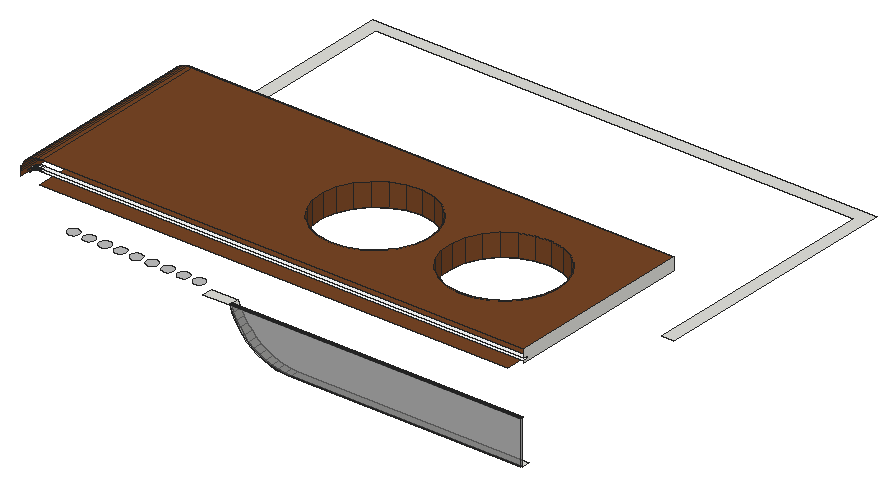
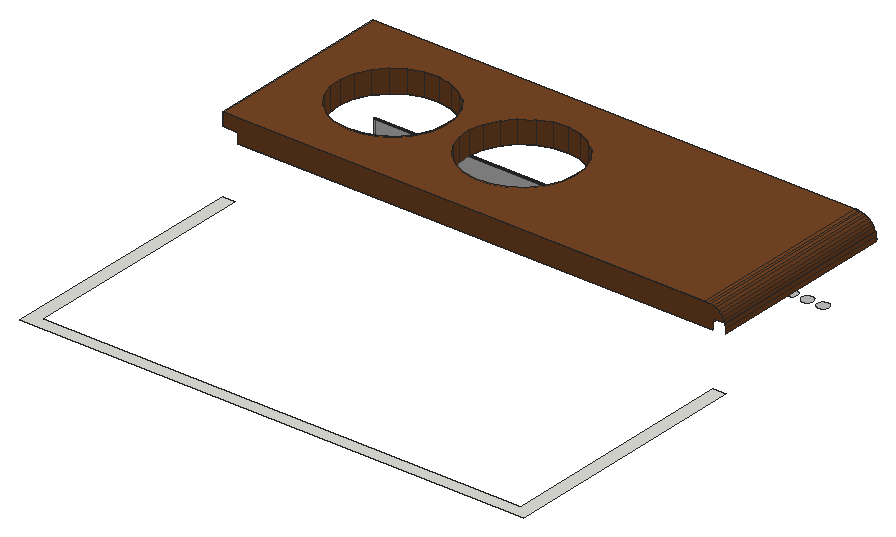
# SketchUp Ruby script. Lengths in millimetres.
U = 1.mm
M = Sketchup.active_model
def pt(a) = Geom::Point3d.new(a.map { |v| v * U })
def face(e, loops, mat)
  f = e.add_face(loops[0].map { |a| pt(a) })
  loops[1..].each { |l| e.add_face(l.map { |a| pt(a) }).erase! }
  f.material = f.back_material = mat if mat
  f
end
# faces: each face lists its corners as indices into pts; further lists are holes
def faces(e, pts, list, mat = nil) = list.each { |f| face(e, (f[0].is_a?(Array) ? f : [f]).map { |l| l.map { |i| pts[i] } }, mat) }
# xy, xz, yz: faces in a plane at the given z, y or x. An outline is a flat list of corners, or four numbers for a rectangle; further outlines are holes
def ring(l) = l.size == 4 ? [[l[0], l[1]], [l[2], l[1]], [l[2], l[3]], [l[0], l[3]]] : l.each_slice(2).to_a
def flat(e, list, mat, &to3) = list.each { |f| face(e, (f[0].is_a?(Array) ? f : [f]).map { |l| ring(l).map { |u, v| to3.(u, v) } }, mat) }
def xy(e, z, list, mat = nil) = flat(e, list, mat) { |x, y| [x, y, z] }
def xz(e, y, list, mat = nil) = flat(e, list, mat) { |x, z| [x, y, z] }
def yz(e, x, list, mat = nil) = flat(e, list, mat) { |y, z| [x, y, z] }
def lines(e, pts, list) = list.each { |a, b| e.add_line(pt(pts[a]), pt(pts[b])) }
# prism: a flat outline (further loops are holes) pulled along v
def prism(e, loops, v, mat = nil)
  f = face(e, loops, mat); d = Geom::Vector3d.new(v.map { |x| x * U })
  f.pushpull(f.normal.samedirection?(d) ? d.length : -d.length)
end
def box(e, o, s, mat = nil) = prism(e, [[o, [o[0] + s[0], o[1], o[2]], [o[0] + s[0], o[1] + s[1], o[2]], [o[0], o[1] + s[1], o[2]]]], [0, 0, s[2]], mat)
def at(x, y, z, deg = 0) = Geom::Transformation.translation(pt([x, y, z])) * Geom::Transformation.rotation(ORIGIN, Z_AXIS, deg.degrees)
def axes(o, x, y, z) = Geom::Transformation.new([*x, 0, *y, 0, *z, 0, *pt(o).to_a, 1])
def part(name) = M.definitions.add(name)
# library, detail: a bought-in or finely detailed component or shape, given as its bounding box
def library(name, o, s) = part(name).tap { |d| box(d.entities, o, s) }
def detail(e, o, s) = box(e.add_group.entities, o, s)
def put(e, d, t, mat = nil) = e.add_instance(d, t).tap { |i| i.material = mat if mat }
def group(e, t, mat = nil) = e.add_group.tap { |g| g.transformation = t; g.material = mat if mat }.entities
root = M.entities
M.materials.add("[Color M00]").color = [255, 255, 255]
M.materials.add("[Color M07]").color = [58, 58, 58]
M.materials.add("[Metal Corrugated Shiny]").color = [193, 193, 193]
M.materials.add("[Translucent Glass Gray]").color = [128, 128, 128]
M.materials["[Translucent Glass Gray]"].alpha = 0.5
M.materials.add("[Wood Veneer 01]").color = [120, 70, 37]
xy(root,7765.4,[[6213.6,642.9,11814.3,849.3]])
xy(root,7765.4,[[6213.6,582.5,11814.3,606.3],[6213.6,606.3,11814.3,642.9]],"[Translucent Glass Gray]")
xy(root,8813.8,[[4124.5,582.5,4764.3,849.3],[3.3,4760.9,308.1,4760.9,308.1,10572.8,11890.5,10572.8,11890.5,4760.9,12195.3,4760.9,12195.3,10877.6,3.3,10877.6]])
xy(root,8813.8,[[4764.3,606.3,11814.3,642.9]],"[Color M07]")
xy(root,8813.8,[[696.7,818.4,730.8,823.2,762.4,836.7,789.5,858,810.2,885.5,823,917.4,827.1,951.5,822.3,985.6,808.8,1017.2,787.6,1044.3,760.1,1064.9,728.2,1077.8,694,1081.9,660,1077.1,628.3,1063.6,601.3,1042.4,580.6,1014.9,567.8,983,563.6,948.8,568.5,914.8,582,883.1,603.2,856,630.7,835.4,662.6,822.5],[1077.7,818.4,1111.8,823.2,1143.4,836.7,1170.5,858,1191.2,885.5,1204,917.4,1208.1,951.5,1203.3,985.6,1189.8,1017.2,1168.6,1044.3,1141.1,1064.9,1109.2,1077.8,1075,1081.9,1041,1077.1,1009.3,1063.6,982.3,1042.4,961.6,1014.9,948.8,983,944.6,948.8,949.5,914.8,963,883.1,984.2,856,1011.7,835.4,1043.6,822.5],[1458.7,818.4,1492.8,823.2,1524.4,836.7,1551.5,858,1572.2,885.5,1585,917.4,1589.1,951.5,1584.3,985.6,1570.8,1017.2,1549.6,1044.3,1522.1,1064.9,1490.2,1077.8,1456,1081.9,1422,1077.1,1390.3,1063.6,1363.3,1042.4,1342.6,1014.9,1329.8,983,1325.6,948.8,1330.5,914.8,1344,883.1,1365.2,856,1392.7,835.4,1424.6,822.5],[1839.7,818.4,1873.8,823.2,1905.4,836.7,1932.5,858,1953.2,885.5,1966,917.4,1970.1,951.5,1965.3,985.6,1951.8,1017.2,1930.6,1044.3,1903.1,1064.9,1871.2,1077.8,1837,1081.9,1803,1077.1,1771.3,1063.6,1744.3,1042.4,1723.6,1014.9,1710.8,983,1706.6,948.8,1711.5,914.8,1725,883.1,1746.2,856,1773.7,835.4,1805.6,822.5],[2220.7,818.4,2254.8,823.2,2286.4,836.7,2313.5,858,2334.2,885.5,2347,917.4,2351.1,951.5,2346.3,985.6,2332.8,1017.2,2311.6,1044.3,2284.1,1064.9,2252.2,1077.8,2218,1081.9,2184,1077.1,2152.3,1063.6,2125.3,1042.4,2104.6,1014.9,2091.8,983,2087.6,948.8,2092.5,914.8,2106,883.1,2127.2,856,2154.7,835.4,2186.6,822.5],
  [2601.7,818.4,2635.8,823.2,2667.4,836.7,2694.5,858,2715.2,885.5,2728,917.4,2732.1,951.5,2727.3,985.6,2713.8,1017.2,2692.6,1044.3,2665.1,1064.9,2633.2,1077.8,2599,1081.9,2565,1077.1,2533.3,1063.6,2506.3,1042.4,2485.6,1014.9,2472.8,983,2468.6,948.8,2473.5,914.8,2487,883.1,2508.2,856,2535.7,835.4,2567.6,822.5],[2982.7,818.4,3016.8,823.2,3048.4,836.7,3075.5,858,3096.2,885.5,3109,917.4,3113.1,951.5,3108.3,985.6,3094.8,1017.2,3073.6,1044.3,3046.1,1064.9,3014.2,1077.8,2980,1081.9,2946,1077.1,2914.3,1063.6,2887.3,1042.4,2866.6,1014.9,2853.8,983,2849.6,948.8,2854.5,914.8,2868,883.1,2889.2,856,2916.7,835.4,2948.6,822.5],[3363.7,818.4,3397.8,823.2,3429.4,836.7,3456.5,858,3477.2,885.5,3490,917.4,3494.1,951.5,3489.3,985.6,3475.8,1017.2,3454.6,1044.3,3427.1,1064.9,3395.2,1077.8,3361,1081.9,3327,1077.1,3295.3,1063.6,3268.3,1042.4,3247.6,1014.9,3234.8,983,3230.6,948.8,3235.5,914.8,3249,883.1,3270.2,856,3297.7,835.4,3329.6,822.5],[3744.7,818.4,3778.8,823.2,3810.4,836.7,3837.5,858,3858.2,885.5,3871,917.4,3875.1,951.5,3870.3,985.6,3856.8,1017.2,3835.6,1044.3,3808.1,1064.9,3776.2,1077.8,3742,1081.9,3708,1077.1,3676.3,1063.6,3649.3,1042.4,3628.6,1014.9,3615.8,983,3611.6,948.8,3616.5,914.8,3630,883.1,3651.2,856,3678.7,835.4,3710.6,822.5]],"[Metal Corrugated Shiny]")
xy(root,8839.2,[[4764.3,606.3,11814.3,642.9]],"[Color M07]")
xy(root,10096.5,[[[479.5,209.6,11814.3,4760.9],[9848.2,1135,10193.1,1163.4,10518.9,1280.1,10803.4,1477.1,11027.2,1741,11175.1,2053.9,11236.9,2394.3,11208.5,2739.2,11091.9,3065,10894.9,3349.5,10630.9,3573.3,10318.1,3721.2,9977.6,3783,9632.7,3754.6,9307,3638,9022.5,3441,8798.7,3177,8650.8,2864.2,8588.9,2523.7,8617.3,2178.8,8734,1853.1,8931,1568.6,9194.9,1344.8,9507.8,1196.9],[6725.6,1135,7070.5,1163.4,7396.3,1280.1,7680.8,1477.1,7904.6,1741,8052.4,2053.9,8114.3,2394.3,8085.9,2739.2,7969.3,3065,7772.3,3349.5,7508.3,3573.3,7195.5,3721.2,6855,3783,6510.1,3754.6,6184.4,3638,5899.9,3441,5676.1,3177,5528.2,2864.2,5466.3,2523.7,5494.7,2178.8,5611.4,1853.1,5808.4,1568.6,6072.3,1344.8,6385.2,1196.9]]],"[Wood Veneer 01]")
xy(root,10388.1,[[531,209.6,12195.3,325.4]],"[Color M00]")
xy(root,10446.7,[[531,209.6,12195.3,325.4]],"[Color M00]")
xy(root,10642.6,[[432,209.6,511.9,4760.9],[[511.9,209.6,12195.3,4760.9],[6725.6,1135,6385.2,1196.9,6072.3,1344.8,5808.4,1568.6,5611.4,1853.1,5494.7,2178.8,5466.3,2523.7,5528.2,2864.2,5676.1,3177,5899.9,3441,6184.4,3638,6510.1,3754.6,6855,3783,7195.5,3721.2,7508.3,3573.3,7772.3,3349.5,7969.3,3065,8085.9,2739.2,8114.3,2394.3,8052.4,2053.9,7904.6,1741,7680.8,1477.1,7396.3,1280.1,7070.5,1163.4],[9848.2,1135,9507.8,1196.9,9194.9,1344.8,8931,1568.6,8734,1853.1,8617.3,2178.8,8588.9,2523.7,8650.8,2864.2,8798.7,3177,9022.5,3441,9307,3638,9632.7,3754.6,9977.6,3783,10318.1,3721.2,10630.9,3573.3,10894.9,3349.5,11091.9,3065,11208.5,2739.2,11236.9,2394.3,11175.1,2053.9,11027.2,1741,10803.4,1477.1,10518.9,1280.1,10193.1,1163.4]]],"[Wood Veneer 01]")
xz(root,209.6,[[3.3,10119.6,3.3,10221.2,0,10189.2],[432,10642.6,511.9,10642.6,442.3,10643.9]])
xz(root,606.3,[[4764.3,8813.8,11814.3,8839.2]],"[Color M07]")
xz(root,606.3,[[6213.6,7765.4,11814.3,7765.4,11814.3,8813.8,4764.3,8813.8,4822,8665.4,4894.7,8523.8,4981.9,8390.6,5082.4,8267.2,5195.3,8154.9,5319.2,8055,5452.9,7968.5,5594.8,7896.5,5743.5,7839.6,5897.3,7798.5,6054.6,7773.7]],"[Translucent Glass Gray]")
xz(root,642.9,[[4764.3,8813.8,11814.3,8839.2]],"[Color M07]")
xz(root,642.9,[[6213.6,7765.4,6054.6,7773.7,5897.3,7798.5,5743.5,7839.6,5594.8,7896.5,5452.9,7968.5,5319.2,8055,5195.3,8154.9,5082.4,8267.2,4981.9,8390.6,4894.7,8523.8,4822,8665.4,4764.3,8813.8,11814.3,8813.8,11814.3,7765.4]],"[Translucent Glass Gray]")
xz(root,4760.9,[[3.3,10221.2,3.3,10337.8,29.4,10337.8,24.3,10325.9,7.1,10258.4]])
xz(root,4760.9,[[308.1,10096.5,308.1,10337.8,29.4,10337.8,51.4,10390.1,87.7,10449.5,132.4,10502.9,184.5,10549,242.9,10587,306.3,10615.8,373.3,10634.9,432,10642.6,12195.3,10642.6,12195.3,10337.8,11814.3,10337.8,11814.3,10096.5]],"[Wood Veneer 01]")
yz(root,3.3,[[209.6,10119.6,4760.9,10221.2],[209.6,10221.2,4760.9,10337.8]],"[Wood Veneer 01]")
yz(root,4764.3,[[606.3,8813.8,642.9,8839.2]],"[Color M07]")
yz(root,11814.3,[[606.3,8813.8,642.9,8839.2]],"[Color M07]")
yz(root,11814.3,[[606.3,7765.4,642.9,8813.8]],"[Translucent Glass Gray]")
yz(root,12195.3,[[209.6,10337.8,4760.9,10337.8,4760.9,10642.6,209.6,10642.6,209.6,10446.7,325.4,10446.7,325.4,10388.1,209.6,10388.1]])
p = [[6054.6,582.5,7773.7],[6213.6,582.5,7765.4],[6213.6,606.3,7765.4],[6054.6,606.3,7773.7],[6054.6,642.9,7773.7],[6213.6,642.9,7765.4],
  [6054.6,849.3,7773.7],[6213.6,849.3,7765.4],[5897.3,582.5,7798.5],[5897.3,606.3,7798.5],[5897.3,642.9,7798.5],[5897.3,849.3,7798.5],
  [5743.5,582.5,7839.6],[5743.5,606.3,7839.6],[5743.5,642.9,7839.6],[5743.5,849.3,7839.6],[5594.8,582.5,7896.5],[5594.8,606.3,7896.5],
  [5594.8,642.9,7896.5],[5594.8,849.3,7896.5],[5452.9,582.5,7968.5],[5452.9,606.3,7968.5],[5452.9,642.9,7968.5],[5452.9,849.3,7968.5],
  [5319.2,582.5,8055],[5319.2,606.3,8055],[5319.2,642.9,8055],[5319.2,849.3,8055],[5195.3,582.5,8154.9],[5195.3,606.3,8154.9],
  [5195.3,642.9,8154.9],[5195.3,849.3,8154.9],[5082.4,582.5,8267.2],[5082.4,606.3,8267.2],[5082.4,642.9,8267.2],[5082.4,849.3,8267.2],
  [4981.9,582.5,8390.6],[4981.9,606.3,8390.6],[4981.9,642.9,8390.6],[4981.9,849.3,8390.6],[4894.7,582.5,8523.8],[4894.7,606.3,8523.8],
  [4894.7,642.9,8523.8],[4894.7,849.3,8523.8],[4822,582.5,8665.4],[4822,606.3,8665.4],[4822,642.9,8665.4],[4822,849.3,8665.4],
  [4764.3,582.5,8813.8],[4764.3,606.3,8813.8],[4764.3,642.9,8813.8],[4764.3,849.3,8813.8],[6385.2,1196.9,10642.6],[6725.6,1135,10642.6],
  [6725.6,1135,10096.5],[6385.2,1196.9,10096.5],[7070.5,1163.4,10642.6],[7070.5,1163.4,10096.5],[9507.8,1196.9,10642.6],[9848.2,1135,10642.6],
  [9848.2,1135,10096.5],[9507.8,1196.9,10096.5],[10193.1,1163.4,10642.6],[10193.1,1163.4,10096.5],[7396.3,1280.1,10642.6],[7396.3,1280.1,10096.5],
  [10518.9,1280.1,10642.6],[10518.9,1280.1,10096.5],[6072.3,1344.8,10642.6],[6072.3,1344.8,10096.5],[9194.9,1344.8,10642.6],[9194.9,1344.8,10096.5],
  [7680.8,1477.1,10642.6],[7680.8,1477.1,10096.5],[10803.4,1477.1,10642.6],[10803.4,1477.1,10096.5],[5808.4,1568.6,10642.6],[5808.4,1568.6,10096.5],
  [8931,1568.6,10642.6],[8931,1568.6,10096.5],[7904.6,1741,10642.6],[7904.6,1741,10096.5],[11027.2,1741,10642.6],[11027.2,1741,10096.5],
  [5611.4,1853.1,10642.6],[5611.4,1853.1,10096.5],[8734,1853.1,10642.6],[8734,1853.1,10096.5],[8052.4,2053.9,10642.6],[8052.4,2053.9,10096.5],
  [11175.1,2053.9,10642.6],[11175.1,2053.9,10096.5],[5494.7,2178.8,10642.6],[5494.7,2178.8,10096.5],[8617.3,2178.8,10642.6],[8617.3,2178.8,10096.5],
  [8114.3,2394.3,10642.6],[8114.3,2394.3,10096.5],[11236.9,2394.3,10642.6],[11236.9,2394.3,10096.5],[5466.3,2523.7,10642.6],[5466.3,2523.7,10096.5],
  [8588.9,2523.7,10642.6],[8588.9,2523.7,10096.5],[8085.9,2739.2,10642.6],[8085.9,2739.2,10096.5],[11208.5,2739.2,10642.6],[11208.5,2739.2,10096.5],
  [5528.2,2864.2,10642.6],[5528.2,2864.2,10096.5],[8650.8,2864.2,10642.6],[8650.8,2864.2,10096.5],[7969.3,3065,10642.6],[7969.3,3065,10096.5],
  [11091.9,3065,10642.6],[11091.9,3065,10096.5],[5676.1,3177,10642.6],[5676.1,3177,10096.5],[8798.7,3177,10642.6],[8798.7,3177,10096.5],
  [7772.3,3349.5,10642.6],[7772.3,3349.5,10096.5],[10894.9,3349.5,10642.6],[10894.9,3349.5,10096.5],[5899.9,3441,10642.6],[5899.9,3441,10096.5],
  [9022.5,3441,10642.6],[9022.5,3441,10096.5],[7508.3,3573.3,10642.6],[7508.3,3573.3,10096.5],[10630.9,3573.3,10642.6],[10630.9,3573.3,10096.5],
  [6184.4,3638,10642.6],[6184.4,3638,10096.5],[9307,3638,10642.6],[9307,3638,10096.5],[7195.5,3721.2,10642.6],[7195.5,3721.2,10096.5],
  [10318.1,3721.2,10642.6],[10318.1,3721.2,10096.5],[6510.1,3754.6,10642.6],[6510.1,3754.6,10096.5],[9632.7,3754.6,10642.6],[9632.7,3754.6,10096.5],
  [6855,3783,10642.6],[6855,3783,10096.5],[9977.6,3783,10642.6],[9977.6,3783,10096.5],[3.3,209.6,10221.2],[7.1,209.6,10258.4],
  [7.1,4760.9,10258.4],[3.3,4760.9,10221.2],[24.3,209.6,10325.9],[24.3,4760.9,10325.9],[241.3,209.6,10274.1],[257,209.6,10297.2],
  [257,325.4,10297.2],[241.3,325.4,10274.1],[275,209.6,10318.5],[275,325.4,10318.5],[202.4,209.6,10329.9],[181.8,209.6,10303.9],
  [181.8,325.4,10303.9],[202.4,325.4,10329.9],[295.2,209.6,10337.7],[295.2,325.4,10337.7],[51.4,209.6,10390.1],[51.4,4760.9,10390.1],
  [29.4,4760.9,10337.8],[219.1,209.6,10347.4],[219.1,325.4,10347.4],[317.5,209.6,10354.5],[317.5,325.4,10354.5],[225.2,209.6,10353.9],
  [225.2,325.4,10353.9],[250.2,209.6,10375.7],[250.2,325.4,10375.7],[341.4,209.6,10368.8],[341.4,325.4,10368.8],[366.8,209.6,10380.4],
  [366.8,325.4,10380.4],[277.2,209.6,10395],[277.2,325.4,10395],[393.2,209.6,10389.2],[393.2,325.4,10389.2],[503.8,209.6,10394.3],
  [531,209.6,10388.1],[531,325.4,10388.1],[503.8,325.4,10394.3],[420.5,209.6,10395],[420.5,325.4,10395],[87.7,209.6,10449.5],
  [87.7,4760.9,10449.5],[476.2,209.6,10397.6],[476.2,325.4,10397.6],[305.8,209.6,10411.7],[305.8,325.4,10411.7],[448.3,209.6,10397.9],
  [448.3,325.4,10397.9],[335.8,209.6,10425.7],[335.8,325.4,10425.7],[367.1,209.6,10436.8],[367.1,325.4,10436.8],[399.2,209.6,10444.9],
  [399.2,325.4,10444.9],[431.9,209.6,10450],[431.9,325.4,10450],[531,209.6,10446.7],[498.1,209.6,10450.9],[498.1,325.4,10450.9],
  [531,325.4,10446.7],[132.4,209.6,10502.9],[132.4,4760.9,10502.9],[465,209.6,10452],[465,325.4,10452],[184.5,209.6,10549],
  [184.5,4760.9,10549],[242.9,209.6,10587],[242.9,4760.9,10587],[306.3,209.6,10615.8],[306.3,4760.9,10615.8],[373.3,209.6,10634.9],
  [373.3,4760.9,10634.9],[432,209.6,10642.6],[432,4760.9,10642.6]]
faces(root,p,[[0,1,2,3],[4,3,2,5],[8,0,3,9],[10,9,3,4],[12,8,9,13],[14,13,9,10],[16,12,13,17],[18,17,13,14],
  [20,16,17,21],[22,21,17,18],[24,20,21,25],[26,25,21,22],[28,24,25,29],[30,29,25,26],[32,28,29,33],[34,33,29,30],
  [36,32,33,37],[38,37,33,34],[40,36,37,41],[42,41,37,38],[44,40,41,45],[46,45,41,42],[48,44,45,49],[50,49,45,46]],"[Translucent Glass Gray]")
faces(root,p,[[6,4,5,7],[11,10,4,6],[15,14,10,11],[19,18,14,15],[23,22,18,19],[27,26,22,23],[31,30,26,27],[35,34,30,31],
  [39,38,34,35],[43,42,38,39],[47,46,42,43],[51,50,46,47]])
faces(root,p,[[52,53,54,55],[53,56,57,54],[58,59,60,61],[59,62,63,60],[56,64,65,57],[62,66,67,63],[68,52,55,69],[70,58,61,71],
  [64,72,73,65],[66,74,75,67],[76,68,69,77],[78,70,71,79],[72,80,81,73],[74,82,83,75],[84,76,77,85],[86,78,79,87],
  [80,88,89,81],[82,90,91,83],[92,84,85,93],[94,86,87,95],[88,96,97,89],[90,98,99,91],[100,92,93,101],[102,94,95,103],
  [96,104,105,97],[98,106,107,99],[108,100,101,109],[110,102,103,111],[104,112,113,105],[106,114,115,107],[116,108,109,117],[118,110,111,119],
  [112,120,121,113],[114,122,123,115],[124,116,117,125],[126,118,119,127],[120,128,129,121],[122,130,131,123],[132,124,125,133],[134,126,127,135],
  [128,136,137,129],[130,138,139,131],[140,132,133,141],[142,134,135,143],[136,144,145,137],[138,146,147,139],[144,140,141,145],[146,142,143,147],
  [148,149,150,151],[149,152,153,150],[152,166,167,168,153],[166,191,192,167],[191,211,212,192],[211,215,216,212],[215,217,218,216],[217,219,220,218],
  [219,221,222,220],[221,223,224,222]],"[Wood Veneer 01]")
faces(root,p,[[154,155,156,157],[155,158,159,156],[160,161,162,163],[158,164,165,159],[169,160,163,170],[164,171,172,165],[173,169,170,174],[175,173,174,176],
  [171,177,178,172],[177,179,180,178],[181,175,176,182],[179,183,184,180],[185,186,187,188],[183,189,190,184],[193,185,188,194],[195,181,182,196],
  [189,197,198,190],[197,193,194,198],[199,195,196,200],[201,199,200,202],[203,201,202,204],[205,203,204,206],[207,208,209,210],[213,205,206,214],
  [208,213,214,209]],"[Color M00]")
